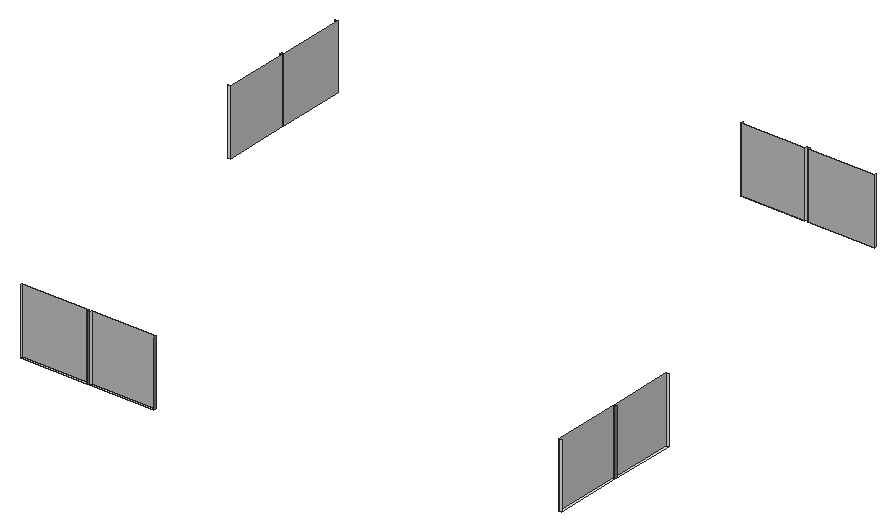
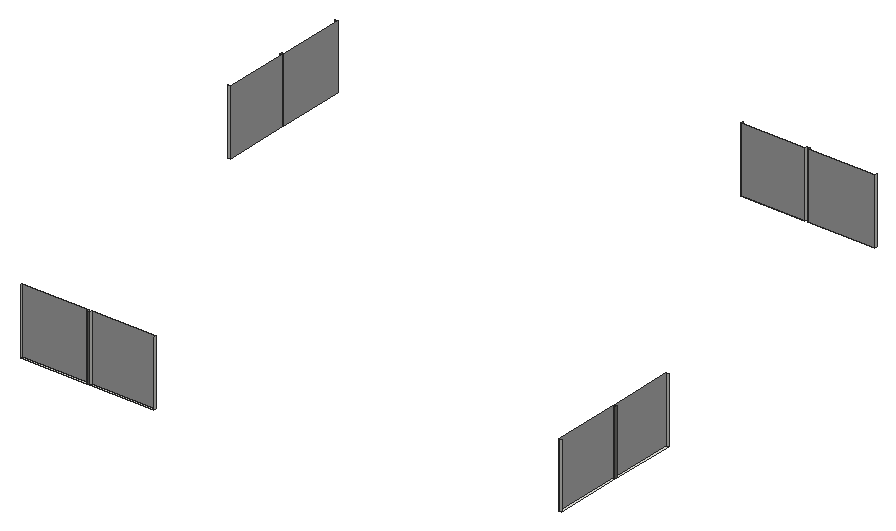
# SketchUp Ruby script. Lengths in inches.
U = 1.inch
M = Sketchup.active_model
def pt(a) = Geom::Point3d.new(a.map { |v| v * U })
def face(e, loops, mat)
  f = e.add_face(loops[0].map { |a| pt(a) })
  loops[1..].each { |l| e.add_face(l.map { |a| pt(a) }).erase! }
  f.material = f.back_material = mat if mat
  f
end
# faces: each face lists its corners as indices into pts; further lists are holes
def faces(e, pts, list, mat = nil) = list.each { |f| face(e, (f[0].is_a?(Array) ? f : [f]).map { |l| l.map { |i| pts[i] } }, mat) }
# xy, xz, yz: faces in a plane at the given z, y or x. An outline is a flat list of corners, or four numbers for a rectangle; further outlines are holes
def ring(l) = l.size == 4 ? [[l[0], l[1]], [l[2], l[1]], [l[2], l[3]], [l[0], l[3]]] : l.each_slice(2).to_a
def flat(e, list, mat, &to3) = list.each { |f| face(e, (f[0].is_a?(Array) ? f : [f]).map { |l| ring(l).map { |u, v| to3.(u, v) } }, mat) }
def xy(e, z, list, mat = nil) = flat(e, list, mat) { |x, y| [x, y, z] }
def xz(e, y, list, mat = nil) = flat(e, list, mat) { |x, z| [x, y, z] }
def yz(e, x, list, mat = nil) = flat(e, list, mat) { |y, z| [x, y, z] }
def lines(e, pts, list) = list.each { |a, b| e.add_line(pt(pts[a]), pt(pts[b])) }
# prism: a flat outline (further loops are holes) pulled along v
def prism(e, loops, v, mat = nil)
  f = face(e, loops, mat); d = Geom::Vector3d.new(v.map { |x| x * U })
  f.pushpull(f.normal.samedirection?(d) ? d.length : -d.length)
end
def box(e, o, s, mat = nil) = prism(e, [[o, [o[0] + s[0], o[1], o[2]], [o[0] + s[0], o[1] + s[1], o[2]], [o[0], o[1] + s[1], o[2]]]], [0, 0, s[2]], mat)
def at(x, y, z, deg = 0) = Geom::Transformation.translation(pt([x, y, z])) * Geom::Transformation.rotation(ORIGIN, Z_AXIS, deg.degrees)
def axes(o, x, y, z) = Geom::Transformation.new([*x, 0, *y, 0, *z, 0, *pt(o).to_a, 1])
def part(name) = M.definitions.add(name)
# library, detail: a bought-in or finely detailed component or shape, given as its bounding box
def library(name, o, s) = part(name).tap { |d| box(d.entities, o, s) }
def detail(e, o, s) = box(e.add_group.entities, o, s)
def put(e, d, t, mat = nil) = e.add_instance(d, t).tap { |i| i.material = mat if mat }
def group(e, t, mat = nil) = e.add_group.tap { |g| g.transformation = t; g.material = mat if mat }.entities
root = M.entities
M.materials.add("[Metal Seamed]").color = [118, 119, 115]
M.materials.add("[Mirror 01]").color = [185, 185, 185]
xy(root,1619.76,[[312.65,102.8125,473.9375,108.8125],[479.9375,102.8125,635.22,108.8125],[1476,277.47,1482,438.75],[1476,444.75,1482,600.03],[138,949.59,144,1104.875],
  [138,1110.875,144,1272.16],[984.78,1440.8125,1140.0625,1446.8125],[1146.0625,1440.8125,1307.35,1446.8125]])
xz(root,102.8125,[[473.9375,1619.76,479.9375,1776.625]],"[Metal Seamed]")
xz(root,108.8125,[[312.65,1619.76,473.9375,1776.625],[479.9375,1619.76,635.22,1776.625]],"[Mirror 01]")
xz(root,277.47,[[1476,1619.76,1482,1776.625]])
xz(root,438.75,[[1476,1619.76,1482,1776.625]])
xz(root,444.75,[[1476,1619.76,1482,1776.625]])
xz(root,600.03,[[1476,1619.76,1482,1776.625]])
xz(root,949.59,[[138,1619.76,144,1776.625]])
xz(root,1104.875,[[138,1619.76,144,1776.625]])
xz(root,1110.875,[[138,1619.76,144,1776.625]])
xz(root,1272.16,[[138,1619.76,144,1776.625]])
xz(root,1440.8125,[[984.78,1619.76,1140.0625,1776.625],[1146.0625,1619.76,1307.35,1776.625]],"[Mirror 01]")
xz(root,1446.8125,[[1140.0625,1619.76,1146.0625,1776.625]],"[Metal Seamed]")
yz(root,138,[[1104.875,1619.76,1110.875,1776.625]],"[Metal Seamed]")
yz(root,144,[[949.59,1619.76,1104.875,1776.625],[1110.875,1619.76,1272.16,1776.625]],"[Mirror 01]")
yz(root,312.65,[[102.8125,1619.76,108.8125,1776.625]])
yz(root,473.9375,[[102.8125,1619.76,108.8125,1776.625]],"[Metal Seamed]")
yz(root,479.9375,[[102.8125,1619.76,108.8125,1776.625]])
yz(root,635.22,[[102.8125,1619.76,108.8125,1776.625]],"[Metal Seamed]")
yz(root,984.78,[[1440.8125,1619.76,1446.8125,1776.625]])
yz(root,1140.0625,[[1440.8125,1619.76,1446.8125,1776.625]])
yz(root,1146.0625,[[1440.8125,1619.76,1446.8125,1776.625]])
yz(root,1307.35,[[1440.8125,1619.76,1446.8125,1776.625]])
yz(root,1476,[[277.47,1619.76,438.75,1776.625],[444.75,1619.76,600.03,1776.625]],"[Mirror 01]")
yz(root,1482,[[438.75,1619.76,444.75,1776.625]],"[Metal Seamed]")
